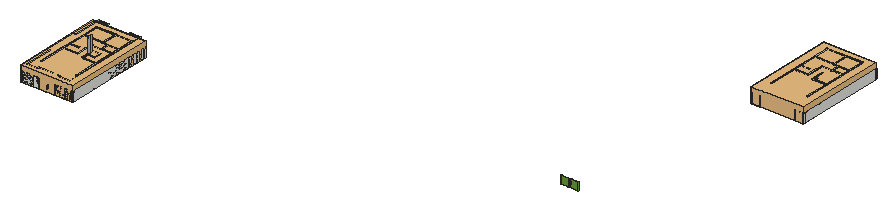
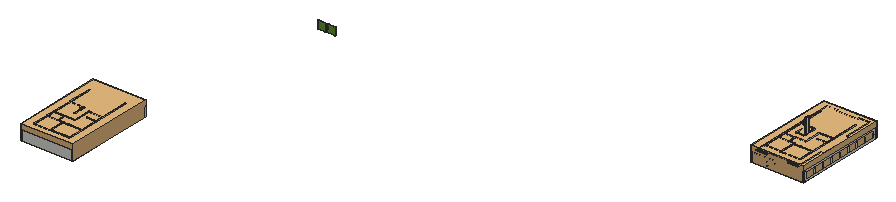
# SketchUp Ruby script. Lengths in inches.
U = 1.inch
M = Sketchup.active_model
def pt(a) = Geom::Point3d.new(a.map { |v| v * U })
def face(e, loops, mat)
  f = e.add_face(loops[0].map { |a| pt(a) })
  loops[1..].each { |l| e.add_face(l.map { |a| pt(a) }).erase! }
  f.material = f.back_material = mat if mat
  f
end
# faces: each face lists its corners as indices into pts; further lists are holes
def faces(e, pts, list, mat = nil) = list.each { |f| face(e, (f[0].is_a?(Array) ? f : [f]).map { |l| l.map { |i| pts[i] } }, mat) }
# xy, xz, yz: faces in a plane at the given z, y or x. An outline is a flat list of corners, or four numbers for a rectangle; further outlines are holes
def ring(l) = l.size == 4 ? [[l[0], l[1]], [l[2], l[1]], [l[2], l[3]], [l[0], l[3]]] : l.each_slice(2).to_a
def flat(e, list, mat, &to3) = list.each { |f| face(e, (f[0].is_a?(Array) ? f : [f]).map { |l| ring(l).map { |u, v| to3.(u, v) } }, mat) }
def xy(e, z, list, mat = nil) = flat(e, list, mat) { |x, y| [x, y, z] }
def xz(e, y, list, mat = nil) = flat(e, list, mat) { |x, z| [x, y, z] }
def yz(e, x, list, mat = nil) = flat(e, list, mat) { |y, z| [x, y, z] }
def lines(e, pts, list) = list.each { |a, b| e.add_line(pt(pts[a]), pt(pts[b])) }
# prism: a flat outline (further loops are holes) pulled along v
def prism(e, loops, v, mat = nil)
  f = face(e, loops, mat); d = Geom::Vector3d.new(v.map { |x| x * U })
  f.pushpull(f.normal.samedirection?(d) ? d.length : -d.length)
end
def box(e, o, s, mat = nil) = prism(e, [[o, [o[0] + s[0], o[1], o[2]], [o[0] + s[0], o[1] + s[1], o[2]], [o[0], o[1] + s[1], o[2]]]], [0, 0, s[2]], mat)
def at(x, y, z, deg = 0) = Geom::Transformation.translation(pt([x, y, z])) * Geom::Transformation.rotation(ORIGIN, Z_AXIS, deg.degrees)
def axes(o, x, y, z) = Geom::Transformation.new([*x, 0, *y, 0, *z, 0, *pt(o).to_a, 1])
def part(name) = M.definitions.add(name)
# library, detail: a bought-in or finely detailed component or shape, given as its bounding box
def library(name, o, s) = part(name).tap { |d| box(d.entities, o, s) }
def detail(e, o, s) = box(e.add_group.entities, o, s)
def put(e, d, t, mat = nil) = e.add_instance(d, t).tap { |i| i.material = mat if mat }
def group(e, t, mat = nil) = e.add_group.tap { |g| g.transformation = t; g.material = mat if mat }.entities
root = M.entities
M.materials.add("0-SS4").color = [255, 255, 255]
M.materials.add("0-SS7").color = [192, 192, 192]
M.materials.add("0-grey 3").color = [204, 204, 204]
M.materials.add("0-off white").color = [255, 255, 255]
M.materials.add("Marble_06_1K").color = [165, 150, 147]
M.materials.add("Tile_Exterior_08_1K1").color = [62, 60, 47]
M.materials.add("[Grass Dark Green]").color = [106, 157, 55]
M.materials.add("polished steel").color = [183, 187, 190]
M.materials.add("steel").color = [179, 179, 179]
c1 = library("Group133\#1",[-5.87,-26.15,0],[281.94,354.24,0.24])
c2 = part("Group\#74")
prism(c2.entities,[[[-5.87,-197.85,-0.61],[-5.87,26.15,-0.61],[-5.87,354.36,-0.61],[282.32,354.36,-0.61],[282.32,-197.85,-0.61]],[[168.74,48.09,-0.61],[228.75,48.09,-0.61],[228.75,108.1,-0.61],[168.74,108.1,-0.61]]],[0,0,0.61])
put(c2.entities,c1,axes([0,20.59,0],[1,0,0],[0,1.01695,0],[0,0,1]))
c3 = part("faewg")
xy(c3.entities,0,[[0,-3,2,0]])
xy(c3.entities,1,[[0,-2,2,0]])
xy(c3.entities,23,[[0,-2,2,0]])
xy(c3.entities,24,[[0,-3,2,0]])
xz(c3.entities,-3,[[0,0,2,24]],"polished steel")
xz(c3.entities,-2,[[0,1,2,23]])
xz(c3.entities,0,[[0,0,2,1],[0,23,2,24]])
yz(c3.entities,0,[[-3,0,-3,24,0,24,0,23,-2,23,-2,1,0,1,0,0]])
yz(c3.entities,2,[[-3,0,0,0,0,1,-2,1,-2,23,0,23,0,24,-3,24]])
c4 = part("reg")
xy(c4.entities,0,[[-8.95,3,59.93,5]])
xy(c4.entities,18,[[51.93,0,53.93,3]],"steel")
xy(c4.entities,19,[[51.93,1,53.93,3]],"steel")
xy(c4.entities,41,[[51.93,1,53.93,3]],"steel")
xy(c4.entities,42,[[51.93,0,53.93,3]],"steel")
xy(c4.entities,61,[[-8.95,3,59.93,5]])
xz(c4.entities,0,[[51.93,18,53.93,42]],"polished steel")
xz(c4.entities,1,[[51.93,19,53.93,41]],"steel")
xz(c4.entities,3,[[[-8.95,0,59.93,61],[51.93,18,53.93,19],[51.93,41,53.93,42]]])
xz(c4.entities,3,[[51.93,18,53.93,19],[51.93,41,53.93,42]],"steel")
xz(c4.entities,5,[[-8.95,0,59.93,61]])
yz(c4.entities,-8.95,[[3,0,5,61]])
yz(c4.entities,51.93,[[0,18,0,42,3,42,3,41,1,41,1,19,3,19,3,18]],"steel")
yz(c4.entities,53.93,[[0,18,3,18,3,19,1,19,1,41,3,41,3,42,0,42]],"steel")
yz(c4.entities,59.93,[[3,0,5,61]])
put(c4.entities,c3,axes([51.93,5.4375,42],[1,0,0],[0,-1,0],[0,0,-1]),"steel")
c5 = library("Group134\#1",[-288.2,-191.85,0],[288.2,191.85,0.24])
c6 = library("Group\#51",[0,0,0],[6.9375,42,86.5])
c7 = library("Group\#2",[0,0,0],[421.11,726.62,120])
c8 = part("Group\#3")
xy(c8.entities,0,[[0,-539.85,6,-315.98],[282.2,-539.85,288.2,-348],[180.12,-348,288.2,-342],[282.19,-342,288.2,-185.89],[6,-321.99,114.08,-315.98],
  [114.08,-321.99,120.08,-315.98],[0,-315.98,6,-255.94],[114.08,-315.98,120.08,-233.93],[0,-255.94,6,-249.9375],[6,-255.94,78.05,-249.9375],
  [0,-249.9375,6,-113.72],[114.08,-185.89,196.13,-179.89],[196.13,-185.89,202.14,-179.89],[202.14,-185.89,288.2,-179.89],[196.13,-179.89,202.14,-149.75],
  [282.19,-179.89,288.2,-119.73],[154.1,-119.73,160.11,-113.72],[196.13,-119.73,282.19,-113.72],[282.19,-119.73,288.2,-113.72],[0,-113.72,6,-107.72],
  [6,-113.72,114.08,-107.72],[150.1,-113.72,154.1,-107.72],[154.1,-113.72,160.11,-107.72],[282.19,-113.72,288.2,12.36],[0,-107.72,6,0],
  [154.1,-107.72,160.11,12.36],[0,0,6,12.36],[0,12.36,6,18.37],[6,12.36,154.1,18.37],[154.1,12.36,160.11,18.37],
  [160.11,12.36,282.19,18.37],[282.19,12.36,288.2,18.37]])
xy(c8.entities,36,[[0,-303.98,6,-267.94],[0,-201.9375,6,-149.72],[282.19,-77.72,288.2,-23.64],[0,-71.72,6,-11.64],[54,12.36,118.1,18.37],
  [196.11,12.36,246.19,18.37]])
xy(c8.entities,84,[[0,-303.98,6,-267.94],[114.08,-233.93,120.08,-185.89],[0,-201.9375,6,-149.72],[196.13,-149.75,202.14,-119.73],[160.11,-119.73,196.13,-113.72],
  [114.08,-113.72,150.1,-107.72],[282.19,-77.72,288.2,-23.64],[0,-71.72,6,-11.64],[54,12.36,118.1,18.37],[196.11,12.36,246.19,18.37]])
xy(c8.entities,96,[[282.19,-161.89,288.2,-137.73]])
xy(c8.entities,108,[[282.19,-161.89,288.2,-137.73]])
xy(c8.entities,120,[[0,-539.85,6,-315.98],[282.2,-539.85,288.2,-348],[180.12,-348,288.2,-342],[282.19,-342,288.2,-185.89],[6,-321.99,114.08,-315.98],
  [114.08,-321.99,120.08,-315.98],[0,-315.98,6,-255.94],[114.08,-315.98,120.08,-233.93],[0,-255.94,6,-249.9375],[6,-255.94,78.05,-249.9375],
  [0,-249.9375,6,-113.72],[114.08,-233.93,120.08,-185.89],[114.08,-185.89,196.13,-179.89],[196.13,-185.89,202.14,-179.89],[202.14,-185.89,288.2,-179.89],
  [196.13,-179.89,202.14,-149.75],[282.19,-179.89,288.2,-119.73],[196.13,-149.75,202.14,-119.73],[154.1,-119.73,160.11,-113.72],[160.11,-119.73,196.13,-113.72],
  [196.13,-119.73,282.19,-113.72],[282.19,-119.73,288.2,-113.72],[0,-113.72,6,-107.72],[6,-113.72,114.08,-107.72],[114.08,-113.72,150.1,-107.72],
  [150.1,-113.72,154.1,-107.72],[154.1,-113.72,160.11,-107.72],[282.19,-113.72,288.2,12.36],[0,-107.72,6,12.36],[154.1,-107.72,160.11,12.36],
  [0,12.36,6,18.37],[6,12.36,154.1,18.37],[154.1,12.36,160.11,18.37],[160.11,12.36,282.19,18.37],[282.19,12.36,288.2,18.37]])
xz(c8.entities,-539.85,[[0,0,6,120],[282.2,0,288.2,120]])
xz(c8.entities,-348,[[180.12,0,282.2,120],[282.2,0,288.2,120]])
xz(c8.entities,-342,[[180.12,0,282.19,120],[282.19,0,288.2,120]])
xz(c8.entities,-321.99,[[6,0,114.08,120],[114.08,0,120.08,120]])
xz(c8.entities,-315.98,[[0,0,6,120],[6,0,114.08,120],[114.08,0,120.08,120]])
xz(c8.entities,-303.98,[[0,36,6,84]])
xz(c8.entities,-267.94,[[0,36,6,84]])
xz(c8.entities,-255.94,[[0,0,6,120],[6,0,78.05,120]])
xz(c8.entities,-249.9375,[[0,0,6,120],[6,0,78.05,120]])
xz(c8.entities,-233.93,[[114.08,0,120.08,84],[114.08,84,120.08,120]])
xz(c8.entities,-201.9375,[[0,36,6,84]])
xz(c8.entities,-185.89,[[114.08,0,196.13,0,196.13,120,120.08,120,120.08,84,114.08,84],[196.13,0,202.14,120],[202.14,0,282.19,120],[282.19,0,288.2,120],[114.08,84,120.08,120]])
xz(c8.entities,-179.89,[[114.08,0,196.13,120],[196.13,0,202.14,120],[202.14,0,282.19,120],[282.19,0,288.2,120]])
xz(c8.entities,-161.89,[[282.19,96,288.2,108]])
xz(c8.entities,-149.75,[[196.13,0,202.14,84],[196.13,84,202.14,120]])
xz(c8.entities,-149.72,[[0,36,6,84]])
xz(c8.entities,-137.73,[[282.19,96,288.2,108]])
xz(c8.entities,-119.73,[[154.1,0,160.11,120],[196.13,0,282.19,0,282.19,120,202.14,120,202.14,84,196.13,84],[282.19,0,288.2,120],[160.11,84,196.13,120],[196.13,84,202.14,120]])
xz(c8.entities,-113.72,[[0,0,6,120],[6,0,114.08,120],[150.1,0,154.1,120],[154.1,0,160.11,120],[196.13,0,282.19,120],
  [282.19,0,288.2,120],[114.08,84,150.1,120],[160.11,84,196.13,120]])
xz(c8.entities,-107.72,[[0,0,6,120],[6,0,114.08,120],[150.1,0,154.1,120],[114.08,84,150.1,120]])
xz(c8.entities,-77.72,[[282.19,36,288.2,84]])
xz(c8.entities,-71.72,[[0,36,6,84]])
xz(c8.entities,-23.64,[[282.19,36,288.2,84]])
xz(c8.entities,-11.64,[[0,36,6,84]])
xz(c8.entities,12.36,[[0,0,6,120],[[6,0,154.1,120],[54,36,118.1,84]],[154.1,0,160.11,120],[[160.11,0,282.19,120],[196.11,36,246.19,84]],[282.19,0,288.2,120]])
xz(c8.entities,18.37,[[0,0,6,120],[[6,0,154.1,120],[54,36,118.1,84]],[154.1,0,160.11,120],[[160.11,0,282.19,120],[196.11,36,246.19,84]],[282.19,0,288.2,120]])
yz(c8.entities,0,[[-539.85,0,-315.98,120],[[-315.98,0,-255.94,120],[-303.98,36,-267.94,84]],[-255.94,0,-249.9375,120],[[-249.9375,0,-113.72,120],[-201.9375,36,-149.72,84]],[-113.72,0,-107.72,120],
  [[-107.72,0,0,120],[-71.72,36,-11.64,84]],[0,0,12.36,120],[12.36,0,18.37,120]])
yz(c8.entities,6,[[-539.85,0,-533.85,120],[-533.85,0,-321.99,120],[-321.99,0,-315.98,120],[[-315.98,0,-255.94,120],[-303.98,36,-267.94,84]],[-255.94,0,-249.9375,120],
  [[-249.9375,0,-113.72,120],[-201.9375,36,-149.72,84]],[-113.72,0,-107.72,120],[[-107.72,0,12.36,120],[-71.72,36,-11.64,84]],[12.36,0,18.37,120]])
yz(c8.entities,54,[[12.36,36,18.37,84]])
yz(c8.entities,78.05,[[-255.94,0,-249.9375,120]])
yz(c8.entities,114.08,[[-321.99,0,-315.98,120],[-315.98,0,-233.93,120],[-185.89,0,-179.89,120],[-113.72,0,-107.72,84],[-233.93,84,-185.89,120],
  [-113.72,84,-107.72,120]])
yz(c8.entities,118.1,[[12.36,36,18.37,84]])
yz(c8.entities,120.08,[[-321.99,0,-315.98,120],[-315.98,0,-233.93,120],[-233.93,84,-185.89,120]])
yz(c8.entities,150.1,[[-113.72,0,-107.72,84],[-113.72,84,-107.72,120]])
yz(c8.entities,154.1,[[-119.73,0,-113.72,120],[-113.72,0,-107.72,120],[-107.72,0,12.36,120],[12.36,0,18.37,120]])
yz(c8.entities,160.11,[[-119.73,0,-113.72,84],[-113.72,0,12.36,120],[12.36,0,18.37,120],[-119.73,84,-113.72,120]])
yz(c8.entities,180.12,[[-348,0,-342,120]])
yz(c8.entities,196.11,[[12.36,36,18.37,84]])
yz(c8.entities,196.13,[[-185.89,0,-179.89,120],[-179.89,0,-149.75,120],[-119.73,0,-113.72,84],[-149.75,84,-119.73,120],[-119.73,84,-113.72,120]])
yz(c8.entities,202.14,[[-185.89,0,-179.89,120],[-179.89,0,-149.75,120],[-149.75,84,-119.73,120]])
yz(c8.entities,246.19,[[12.36,36,18.37,84]])
yz(c8.entities,282.19,[[-342,0,-185.89,120],[[-179.89,0,-119.73,120],[-161.89,96,-137.73,108]],[-119.73,0,-113.72,120],[[-113.72,0,12.36,120],[-77.72,36,-23.64,84]],[12.36,0,18.37,120]])
yz(c8.entities,282.2,[[-539.85,0,-533.85,120],[-533.85,0,-348,120]])
yz(c8.entities,288.2,[[-539.85,0,-348,120],[-348,0,-342,120],[-342,0,-185.89,120],[-185.89,0,-179.89,120],[[-179.89,0,-119.73,120],[-161.89,96,-137.73,108]],
  [-119.73,0,-113.72,120],[[-113.72,0,12.36,120],[-77.72,36,-23.64,84]],[12.36,0,18.37,120]])
c9 = part("Group\#59")
box(c9.entities,[0,0,0],[12.01,42.03,6.2])
c10 = part("Lift Door")
g1 = group(c10.entities,at(22.98,-1.97,0))
xy(g1,0,[[-11.49,0,22.98,1.97]],"0-SS7")
xy(g1,81.69,[[-11.49,0,22.98,1.97]],"0-SS7")
xz(g1,0,[[-11.49,0,22.98,81.69]],"0-SS7")
xz(g1,1.97,[[-11.49,0,22.98,81.69]],"0-SS4")
yz(g1,-11.49,[[0,0,1.97,81.69]],"0-SS7")
yz(g1,22.98,[[0,0,1.97,81.69]],"0-SS7")
c11 = part("Group\#83")
put(c11.entities,c10,axes([5.4,10.39,0],[0,0.42899,0],[-0.53123,0,0],[0,0,1.07229]),"0-grey 3")
put(c11.entities,c10,axes([5.4,-4.4,0],[0,0.42899,0],[-0.53123,0,0],[0,0,1.07229]),"0-grey 3")
g2 = group(c11.entities,at(0,44.39,0))
p = [[0,-44.39,88.58],[0,-13.75,88.58],[0,-13.75,0],[0,-44.39,0]]
lines(g2,p,[[0,1],[1,2],[3,0],[2,3]])
g3 = group(c11.entities,at(2.42,30.63,0))
prism(g3,[[[2.98,-30.63,0],[2.98,-30.11,0],[2.98,-30.11,87.6],[2.98,-0.53,87.6],[2.98,-0.53,0],[2.98,0,0],[2.98,0,88.58],[2.98,-30.63,88.58]]],[-5.4,0,0])
c12 = library("Slide Window 5'",[0,-2.02,0],[60,2.02,54])
c13 = part("Group\#60")
box(c13.entities,[0,0,0],[42.03,42.03,6])
c14 = part("Group\#66")
box(c14.entities,[0,0,0],[42.03,12.01,6.2])
c15 = part("Group\#305")
xy(c15.entities,0.81,[[0.28,-0.04,1.69,0]],"0-off white")
xz(c15.entities,-0.04,[[0.28,0.81,1.69,0.81,0.98,1.5]],"0-off white")
xz(c15.entities,0,[[[0.98,0,1.24,0.03,1.48,0.13,1.68,0.29,1.84,0.49,1.93,0.73,1.97,0.98,1.93,1.24,1.84,1.48,1.68,1.68,1.48,1.84,1.24,1.93,0.98,1.97,0.73,1.93,0.49,1.84,0.29,1.68,0.13,1.48,0.03,1.24,0,0.98,0.03,0.73,0.13,0.49,0.29,0.29,0.49,0.13,0.73,0.03],[0.28,0.81,0.98,1.5,1.69,0.81]]],"0-off white")
xz(c15.entities,0.63,[[0.98,0,0.73,0.03,0.49,0.13,0.29,0.29,0.13,0.49,0.03,0.73,0,0.98,0.03,1.24,0.13,1.48,0.29,1.68,0.49,1.84,0.73,1.93,0.98,1.97,1.24,1.93,1.48,1.84,1.68,1.68,1.84,1.48,1.93,1.24,1.97,0.98,1.93,0.73,1.84,0.49,1.68,0.29,1.48,0.13,1.24,0.03]],"0-off white")
p = [[0.49,0.63,0.13],[0.73,0.63,0.03],[0.73,0,0.03],[0.49,0,0.13],[0.98,0.63,0],[0.98,0,0],
  [1.24,0.63,0.03],[1.24,0,0.03],[1.48,0.63,0.13],[1.48,0,0.13],[0.29,0.63,0.29],[0.29,0,0.29],
  [1.68,0.63,0.29],[1.68,0,0.29],[0.13,0.63,0.49],[0.13,0,0.49],[1.84,0.63,0.49],[1.84,0,0.49],
  [0.03,0.63,0.73],[0.03,0,0.73],[1.93,0.63,0.73],[1.93,0,0.73],[0,0.63,0.98],[0,0,0.98],
  [1.97,0.63,0.98],[1.97,0,0.98],[0.98,0,1.5],[0.28,0,0.81],[0.28,-0.04,0.81],[0.98,-0.04,1.5],
  [1.69,0,0.81],[1.69,-0.04,0.81],[0.03,0.63,1.24],[0.03,0,1.24],[1.93,0.63,1.24],[1.93,0,1.24],
  [0.13,0.63,1.48],[0.13,0,1.48],[1.84,0.63,1.48],[1.84,0,1.48],[0.29,0.63,1.68],[0.29,0,1.68],
  [1.68,0.63,1.68],[1.68,0,1.68],[0.49,0.63,1.84],[0.49,0,1.84],[1.48,0.63,1.84],[1.48,0,1.84],
  [0.73,0.63,1.93],[0.73,0,1.93],[1.24,0.63,1.93],[1.24,0,1.93],[0.98,0.63,1.97],[0.98,0,1.97]]
faces(c15.entities,p,[[0,1,2,3],[1,4,5,2],[4,6,7,5],[6,8,9,7],[10,0,3,11],[8,12,13,9],[14,10,11,15],[12,16,17,13],
  [18,14,15,19],[16,20,21,17],[22,18,19,23],[20,24,25,21],[26,27,28,29],[30,26,29,31],[32,22,23,33],[24,34,35,25],
  [36,32,33,37],[34,38,39,35],[40,36,37,41],[38,42,43,39],[44,40,41,45],[42,46,47,43],[48,44,45,49],[46,50,51,47],
  [52,48,49,53],[50,52,53,51]],"0-off white")
c16 = part("Group\#370")
box(c16.entities,[0,0,-0.39],[5.12,10.31,0.39])
g4 = group(c16.entities,at(1.59,1.64,0.22))
put(g4,c15,axes([0,4.49,0],[1,0,0],[0,0,-0.35294],[0,1,0]))
put(g4,c15,axes([0,2,0],[1,0,0],[0,0,-0.35294],[0,-1,0]))
c17 = part("Group\#67")
box(c17.entities,[0,0,0],[42.03,42.03,6])
c18 = part("Group\#71")
box(c18.entities,[0,0,0],[12.01,42.03,5.2])
c19 = library("Group\#46",[0,-0.05,0],[30,2.55,24])
c20 = part("Group\#72")
box(c20.entities,[0,0,0],[12.01,42.03,5.4])
c21 = part("Group\#304")
xy(c21.entities,0,[[0,-0.39,16.57,0]])
xy(c21.entities,0.98,[[0.98,-0.39,15.59,-0.2]])
xy(c21.entities,3.86,[[0.98,-0.39,15.59,-0.2]])
xy(c21.entities,4.84,[[0,-0.39,16.57,0]])
xz(c21.entities,-0.39,[[[0,0,16.57,4.84],[0.98,0.98,15.59,3.86]]])
xz(c21.entities,-0.2,[[0.98,0.98,15.59,3.86]])
xz(c21.entities,0,[[0,0,16.57,4.84]])
yz(c21.entities,0,[[-0.39,0,0,4.84]])
yz(c21.entities,0.98,[[-0.39,0.98,-0.2,3.86]])
yz(c21.entities,15.59,[[-0.39,0.98,-0.2,3.86]])
yz(c21.entities,16.57,[[-0.39,0,0,4.84]])
c22 = part("Group\#73")
box(c22.entities,[0,0,0],[12.01,42.03,7.6])
box(root,[236.19,375.57,108],[6.01,36.03,12])
box(root,[3968.93,3010.75,108],[6,36.02,12])
xy(root,-0.01,[[68.08,118.41,356.28,310.26],[3800.8125,2753.59,4089.01,2945.4375]])
put(root,c2,at(73.95,316.26,-0.01))
put(root,c2,at(3806.6875,2951.44,-0.01))
put(root,c4,axes([155.04,1.14,-0.12],[1,0,0],[0,1,0],[0,0,1.28062]),"[Grass Dark Green]")
put(root,c4,axes([270.05,1.14,-0.12],[-0.91903,0,0],[0,1,0],[0,0,1.28062]),"[Grass Dark Green]")
put(root,c5,at(356.28,310.26,-0.01))
put(root,c5,at(4089.01,2945.4375,-0.01))
g5 = group(root,at(0,717.62,0))
xy(g5,0,[[0,-717.62,9,-708.62],[9,-717.62,146.08,-708.62],[278.28,-717.62,412.11,-708.62],[412.11,-717.62,421.11,-708.62],[0,-708.62,9,0],
  [412.11,-708.62,421.11,0],[0,0,9,9],[9,0,412.11,9],[412.11,0,421.11,9]])
xy(g5,12,[[0,-696.62,4,-690],[0,-684,4,-606],[0,-600,4,-522],[0,-516,4,-438],[0,-432,4,-354],
  [0,-348,4,-270],[0,-264,4,-186],[0,-180,4,-102],[0,-96,4,-12]])
xy(g5,66,[[0,-696.62,4,-690],[0,-684,4,-606],[0,-600,4,-522],[0,-516,4,-438],[0,-432,4,-354],
  [0,-348,4,-270],[0,-264,4,-186],[0,-180,4,-102],[0,-96,4,-12]])
xy(g5,78,[[0,-717.62,9,-708.62],[9,-717.62,146.08,-708.62],[278.28,-717.62,412.11,-708.62],[412.11,-717.62,421.11,-708.62],[0,-708.62,9,0],
  [412.11,-708.62,421.11,0],[0,0,9,9],[9,0,412.11,9],[412.11,0,421.11,9]])
xz(g5,-717.62,[[0,0,9,78],[9,0,146.08,78],[278.28,0,412.11,78],[412.11,0,421.11,78]])
xz(g5,-708.62,[[0,0,9,78],[9,0,146.08,78],[278.28,0,412.11,78],[412.11,0,421.11,78]])
xz(g5,-696.62,[[0,12,4,66]])
xz(g5,-690,[[0,12,4,66]])
xz(g5,-684,[[0,12,4,66]])
xz(g5,-606,[[0,12,4,66]])
xz(g5,-600,[[0,12,4,66]])
xz(g5,-522,[[0,12,4,66]])
xz(g5,-516,[[0,12,4,66]])
xz(g5,-438,[[0,12,4,66]])
xz(g5,-432,[[0,12,4,66]])
xz(g5,-354,[[0,12,4,66]])
xz(g5,-348,[[0,12,4,66]])
xz(g5,-270,[[0,12,4,66]])
xz(g5,-264,[[0,12,4,66]])
xz(g5,-186,[[0,12,4,66]])
xz(g5,-180,[[0,12,4,66]])
xz(g5,-102,[[0,12,4,66]])
xz(g5,-96,[[0,12,4,66]])
xz(g5,-12,[[0,12,4,66]])
xz(g5,0,[[0,0,9,78],[9,0,412.11,78],[412.11,0,421.11,78]])
xz(g5,9,[[0,0,9,78],[9,0,412.11,78],[412.11,0,421.11,78]])
yz(g5,0,[[-717.62,0,-708.62,78],[[-708.62,0,0,78],[-696.62,12,-12,66]],[0,0,9,78],[-690,12,-684,66],[-606,12,-600,66],
  [-522,12,-516,66],[-438,12,-432,66],[-354,12,-348,66],[-270,12,-264,66],[-186,12,-180,66],
  [-102,12,-96,66]])
yz(g5,4,[[-696.62,12,-690,66]])
yz(g5,4,[[-684,12,-606,66],[-600,12,-522,66],[-516,12,-438,66],[-432,12,-354,66],[-348,12,-270,66],
  [-264,12,-186,66],[-180,12,-102,66],[-96,12,-12,66]],"Marble_06_1K")
yz(g5,9,[[-717.62,0,-708.62,78],[-708.62,0,0,78],[0,0,9,78]])
yz(g5,146.08,[[-717.62,0,-708.62,78]])
yz(g5,278.28,[[-717.62,0,-708.62,78]])
yz(g5,412.11,[[-717.62,0,-708.62,78],[-708.62,0,0,78],[0,0,9,78]])
yz(g5,421.11,[[-717.62,0,-708.62,78],[-708.62,0,0,78],[0,0,9,78]])
put(root,c6,axes([264.3,508.52,0],[0.85622,0,0],[0,0.71477,0],[0,0,0.97071]))
put(root,c7,at(0,0,0))
put(root,c8,at(68.08,658.26,0))
put(root,c6,axes([264.21,536.875,0],[0,0.85622,0],[-0.85772,0,0],[0,0,0.97071]))
put(root,c9,at(236.19,430.34,0))
g6 = group(root,at(3732.73,3352.8,0))
xy(g6,0,[[0,-717.62,9,-708.62],[9,-717.62,74.08,-708.62],[350.28,-717.62,412.11,-708.62],[412.11,-717.62,421.11,-708.62],[0,-708.62,9,0],
  [412.11,-708.62,421.11,0],[0,0,9,9],[9,0,412.11,9],[412.11,0,421.11,9]])
xy(g6,78,[[0,-717.62,9,-708.62],[9,-717.62,74.08,-708.62],[350.28,-717.62,412.11,-708.62],[412.11,-717.62,421.11,-708.62],[0,-708.62,9,0],
  [412.11,-708.62,421.11,0],[0,0,9,9],[9,0,412.11,9],[412.11,0,421.11,9]])
xz(g6,-717.62,[[0,0,9,78],[9,0,74.08,78],[350.28,0,412.11,78],[412.11,0,421.11,78]])
xz(g6,-708.62,[[0,0,9,78],[9,0,74.08,78],[350.28,0,412.11,78],[412.11,0,421.11,78]])
xz(g6,0,[[0,0,9,78],[9,0,412.11,78],[412.11,0,421.11,78]])
xz(g6,9,[[0,0,9,78],[9,0,412.11,78],[412.11,0,421.11,78]])
yz(g6,0,[[-717.62,0,-708.62,78],[[-708.62,0,0,78],[-696.62,12,-12,66]],[0,0,9,78],[-696.62,12,-12,66]])
yz(g6,9,[[-717.62,0,-708.62,78],[-708.62,0,0,78],[0,0,9,78]])
yz(g6,74.08,[[-717.62,0,-708.62,78]])
yz(g6,350.28,[[-717.62,0,-708.62,78]])
yz(g6,412.11,[[-717.62,0,-708.62,78],[-708.62,0,0,78],[0,0,9,78]])
yz(g6,421.11,[[-717.62,0,-708.62,78],[-708.62,0,0,78],[0,0,9,78]])
put(root,c6,axes([3997.03,3143.69,0],[0.85622,0,0],[0,0.71477,0],[0,0,0.97071]))
put(root,c7,at(3732.73,2635.18,0))
put(root,c8,at(3800.8125,3293.44,0))
put(root,c6,axes([3996.95,3172.05,0],[0,0.85622,0],[-0.85772,0,0],[0,0,0.97071]))
put(root,c9,at(3968.93,3065.52,0))
g7 = group(root,at(9,676.63,0),"Tile_Exterior_08_1K1")
xy(g7,0,[[0,-667.63,347.2,-558.22],[347.2,-667.63,403.11,-558.22],[0,-558.22,59.08,0],[347.2,-558.22,403.11,0],[0,0,59.08,40.99],
  [59.08,0,347.2,40.99],[347.2,0,347.28,40.99],[347.28,0,403.11,40.99]])
xy(g7,0.3,[[0,-667.63,347.2,-558.22],[347.2,-667.63,403.11,-558.22],[0,-558.22,59.08,0],[347.2,-558.22,403.11,0],[0,0,59.08,40.99],
  [59.08,0,347.2,40.99],[347.2,0,347.28,40.99],[347.28,0,403.11,40.99]])
xz(g7,-667.63,[[0,0,347.2,0.3],[347.2,0,403.11,0.3]])
xz(g7,-558.22,[[0,0,59.08,0.3],[59.08,0,347.2,0.3],[347.2,0,403.11,0.3]])
xz(g7,0,[[0,0,59.08,0.3],[59.08,0,347.2,0.3],[347.2,0,347.28,0.3],[347.28,0,403.11,0.3]])
xz(g7,40.99,[[0,0,59.08,0.3],[59.08,0,347.2,0.3],[347.2,0,347.28,0.3],[347.28,0,403.11,0.3]])
yz(g7,0,[[-667.63,0,-558.22,0.3],[-558.22,0,0,0.3],[0,0,40.99,0.3]])
yz(g7,59.08,[[-558.22,0,0,0.3],[0,0,40.99,0.3]])
yz(g7,347.2,[[-667.63,0,-558.22,0.3],[-558.22,0,0,0.3],[0,0,40.99,0.3]])
yz(g7,347.28,[[0,0,40.99,0.3]])
yz(g7,403.11,[[-667.63,0,-558.22,0.3],[-558.22,0,0,0.3],[0,0,40.99,0.3]])
put(root,c11,axes([236.19,375.57,0],[1,0,0],[0,1.17593,0],[0,0,1.2192]))
put(root,c11,axes([3968.93,3010.75,0],[1,0,0],[0,1.17593,0],[0,0,1.2192]))
put(root,c6,axes([189.82,472.37,0],[-0.85622,0,0],[0,-1.14363,0],[0,0,0.9711]))
put(root,c6,axes([3922.55,3107.55,0],[-0.85622,0,0],[0,-1.14363,0],[0,0,0.9711]))
put(root,c6,axes([218.18,542.88,0.03],[0,0.85622,0],[-0.85772,0,0],[0,0,0.97071]))
put(root,c6,axes([3950.92,3178.06,0.03],[0,0.85622,0],[-0.85772,0,0],[0,0,0.97071]))
put(root,c4,at(3459.39,1087.63,1),"[Grass Dark Green]")
put(root,c4,axes([3579.26,1087.63,1],[-1,0,0],[0,1,0],[0,0,1]),"[Grass Dark Green]")
put(root,c9,at(248.2,430.34,6.2))
put(root,c9,at(3980.9375,3065.52,6.2))
put(root,c9,at(260.21,430.34,12.4))
put(root,c9,at(3992.94,3065.52,12.4))
put(root,c9,at(272.22,430.34,18.6))
put(root,c9,at(4004.95,3065.52,18.6))
put(root,c9,at(284.23,430.34,24.8))
put(root,c9,at(4016.96,3065.52,24.8))
put(root,c9,at(296.24,430.34,31))
put(root,c9,at(4028.97,3065.52,31))
put(root,c12,axes([70.35,586.48,35.94],[0,1.06834,0],[-1.4091,0,0],[0,0,0.88889]))
put(root,c12,axes([3803.09,3221.65,35.94],[0,1.06834,0],[-1.4091,0,0],[0,0,0.88889]))
put(root,c12,axes([122.02,674.22,35.94],[1.06834,0,0],[0,1.4091,0],[0,0,0.88889]))
put(root,c12,axes([3854.75,3309.4,35.94],[1.06834,0,0],[0,1.4091,0],[0,0,0.88889]))
put(root,c12,axes([70.24,456.33,36],[0,0.86536,0],[-1.4091,0,0],[0,0,0.88889]))
put(root,c12,axes([3802.97,3091.5,36],[0,0.86536,0],[-1.4091,0,0],[0,0,0.88889]))
put(root,c12,axes([70.24,354.28,36],[0,0.60068,0],[-1.4091,0,0],[0,0,0.88889]))
put(root,c12,axes([3802.97,2989.46,36],[0,0.60068,0],[-1.4091,0,0],[0,0,0.88889]))
put(root,c12,axes([354.12,634.625,36],[0,-0.89997,0],[1.4091,0,0],[0,0,0.88889]))
put(root,c12,axes([4086.85,3269.8,36],[0,-0.89997,0],[1.4091,0,0],[0,0,0.88889]))
put(root,c12,axes([264.1875,673.47,36.625],[0.83331,0,0],[0,1.4091,0],[0,0,0.88]))
put(root,c12,axes([3996.92,3308.65,36.625],[0.83331,0,0],[0,1.4091,0],[0,0,0.88]))
put(root,c13,at(308.24,430.34,37.2))
put(root,c13,at(4040.98,3065.52,37.2))
put(root,c14,at(308.24,418.33,43.2))
put(root,c14,at(4040.98,3053.51,43.2))
put(root,c14,at(308.24,406.33,49.4))
put(root,c14,at(4040.98,3041.5,49.4))
put(root,c16,axes([236.19,421.93,50.66],[0,-0.53664,0],[0,0,1],[-1.59369,0,0]))
put(root,c16,axes([3968.93,3057.1,50.66],[0,-0.53664,0],[0,0,1],[-1.59369,0,0]))
put(root,c14,at(308.24,394.32,55.6))
put(root,c14,at(4040.98,3029.49,55.6))
put(root,c14,at(308.24,382.31,61.8))
put(root,c14,at(4040.98,3017.49,61.8))
put(root,c14,at(308.24,370.3,68))
put(root,c14,at(4040.98,3005.48,68))
put(root,c14,at(308.24,358.29,74.2))
put(root,c14,at(4040.98,2993.47,74.2))
put(root,c17,at(308.24,316.26,80.4))
put(root,c17,at(4040.98,2951.44,80.4))
put(root,c18,at(296.24,316.26,86.4))
put(root,c18,at(4028.97,2951.44,86.4))
put(root,c18,at(284.23,316.26,91.6))
put(root,c18,at(4016.96,2951.44,91.6))
put(root,c19,axes([352.25,520.54,96],[0,-0.80536,0],[1.27878,0,0],[0,0,0.5]))
put(root,c19,axes([4084.98,3155.71,96],[0,-0.80536,0],[1.27878,0,0],[0,0,0.5]))
put(root,c18,at(272.22,316.26,96.8))
put(root,c18,at(4004.95,2951.44,96.8))
put(root,c18,at(260.21,316.26,102))
put(root,c18,at(3992.94,2951.44,102))
put(root,c20,at(248.2,316.26,107.2))
put(root,c20,at(3980.9375,2951.44,107.2))
put(root,c21,axes([236.19,397.64,111.82],[0,-0.53664,0],[1.51401,0,0],[0,0,1.21]))
put(root,c21,axes([3968.93,3032.82,111.82],[0,-0.53664,0],[1.51401,0,0],[0,0,1.21]))
put(root,c22,at(236.19,316.26,112.4))
put(root,c22,at(3968.93,2951.44,112.4))
g8 = group(root,at(-16.2,37.34,114))
xy(g8,0,[[[42,0,42,228,18,228,18,486,42,486,42,713.93,126,713.93,126,690,294.4,690,294.4,713.93,378.4,713.93,378.4,0,294.4,0,294.4,12,126,12,126,0],[258.4,327,318.4,387]]])
xz(g8,0,[[42,0,126,6],[294.4,0,378.4,6]])
xz(g8,12,[[126,0,294.4,6]])
xz(g8,228,[[18,0,42,6]])
xz(g8,327,[[258.4,0,318.4,7]])
xz(g8,387,[[258.4,0,318.4,7]])
xz(g8,486,[[18,0,42,6]])
xz(g8,690,[[126,0,294.4,6]])
xz(g8,713.93,[[42,0,126,6],[294.4,0,378.4,6]])
yz(g8,18,[[228,0,486,6]])
yz(g8,42,[[0,0,228,6],[486,0,713.93,6]])
yz(g8,126,[[0,0,12,6],[690,0,713.93,6]])
yz(g8,258.4,[[327,0,387,7]])
yz(g8,294.4,[[0,0,12,6],[690,0,713.93,6]])
yz(g8,318.4,[[327,0,387,7]])
yz(g8,378.4,[[0,0,713.93,6]])
put(root,c11,axes([236.2,375.58,119.39],[1,0,0],[0,1.17593,0],[0,0,1.36155]))
